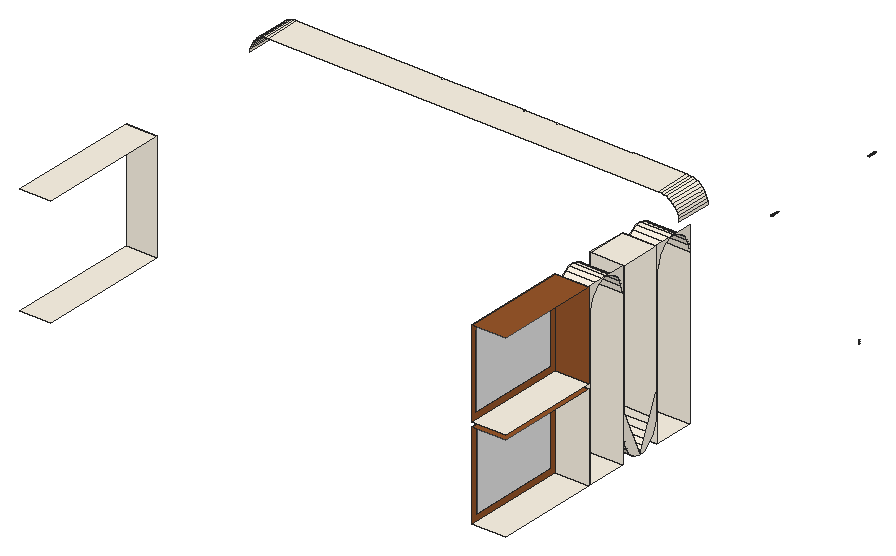
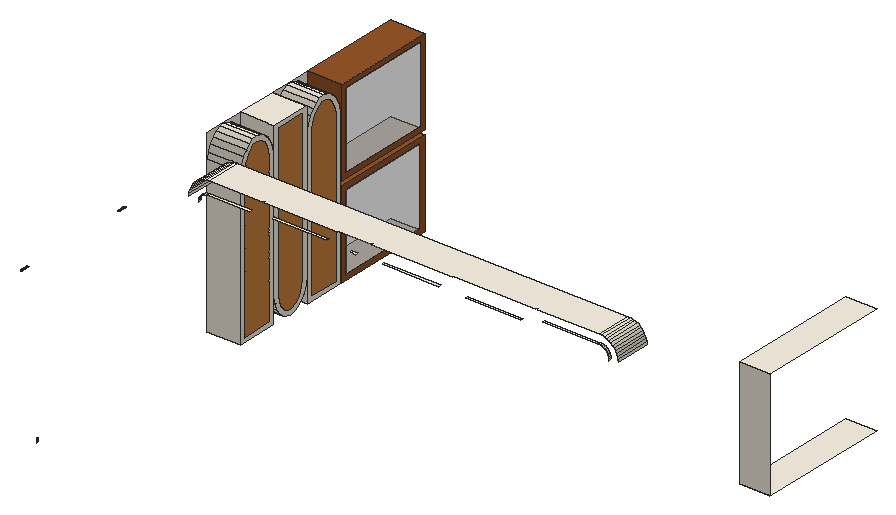
# SketchUp Ruby script. Lengths in inches.
U = 1.inch
M = Sketchup.active_model
def pt(a) = Geom::Point3d.new(a.map { |v| v * U })
def face(e, loops, mat)
  f = e.add_face(loops[0].map { |a| pt(a) })
  loops[1..].each { |l| e.add_face(l.map { |a| pt(a) }).erase! }
  f.material = f.back_material = mat if mat
  f
end
# faces: each face lists its corners as indices into pts; further lists are holes
def faces(e, pts, list, mat = nil) = list.each { |f| face(e, (f[0].is_a?(Array) ? f : [f]).map { |l| l.map { |i| pts[i] } }, mat) }
# xy, xz, yz: faces in a plane at the given z, y or x. An outline is a flat list of corners, or four numbers for a rectangle; further outlines are holes
def ring(l) = l.size == 4 ? [[l[0], l[1]], [l[2], l[1]], [l[2], l[3]], [l[0], l[3]]] : l.each_slice(2).to_a
def flat(e, list, mat, &to3) = list.each { |f| face(e, (f[0].is_a?(Array) ? f : [f]).map { |l| ring(l).map { |u, v| to3.(u, v) } }, mat) }
def xy(e, z, list, mat = nil) = flat(e, list, mat) { |x, y| [x, y, z] }
def xz(e, y, list, mat = nil) = flat(e, list, mat) { |x, z| [x, y, z] }
def yz(e, x, list, mat = nil) = flat(e, list, mat) { |y, z| [x, y, z] }
def lines(e, pts, list) = list.each { |a, b| e.add_line(pt(pts[a]), pt(pts[b])) }
# prism: a flat outline (further loops are holes) pulled along v
def prism(e, loops, v, mat = nil)
  f = face(e, loops, mat); d = Geom::Vector3d.new(v.map { |x| x * U })
  f.pushpull(f.normal.samedirection?(d) ? d.length : -d.length)
end
def box(e, o, s, mat = nil) = prism(e, [[o, [o[0] + s[0], o[1], o[2]], [o[0] + s[0], o[1] + s[1], o[2]], [o[0], o[1] + s[1], o[2]]]], [0, 0, s[2]], mat)
def at(x, y, z, deg = 0) = Geom::Transformation.translation(pt([x, y, z])) * Geom::Transformation.rotation(ORIGIN, Z_AXIS, deg.degrees)
def axes(o, x, y, z) = Geom::Transformation.new([*x, 0, *y, 0, *z, 0, *pt(o).to_a, 1])
def part(name) = M.definitions.add(name)
# library, detail: a bought-in or finely detailed component or shape, given as its bounding box
def library(name, o, s) = part(name).tap { |d| box(d.entities, o, s) }
def detail(e, o, s) = box(e.add_group.entities, o, s)
def put(e, d, t, mat = nil) = e.add_instance(d, t).tap { |i| i.material = mat if mat }
def group(e, t, mat = nil) = e.add_group.tap { |g| g.transformation = t; g.material = mat if mat }.entities
root = M.entities
M.materials.add("Material \#0").color = [86, 53, 35]
M.materials.add("Material \#1").color = [140, 140, 140]
M.materials.add("[0030_OldLace]").color = [253, 245, 230]
M.materials.add("[0040_Peru]").color = [205, 133, 63]
M.materials.add("[Translucent Glass Gray]").color = [128, 128, 128]
M.materials["[Translucent Glass Gray]"].alpha = 0.5
M.materials.add("[Wood Cherry Original]").color = [152, 86, 42]
c1 = part("3DGeom~17_Defintion")
yz(c1.entities,-1908.8,[[-436.03,-21.87,-436.73,-21.5,-435.91,-21.83],[436.03,-21.87,435.91,-21.83,436.73,-21.5],[-435.91,-21.83,-436.73,-21.5,-436.15,-21.125],[-435.91,-21.83,-436.15,-21.125,-435.87,-21.72],[435.91,-21.83,435.87,-21.72,436.15,-21.125],
  [435.91,-21.83,436.15,-21.125,436.73,-21.5],[-436.73,-21.5,-484.73,-21.37,-436.15,-1.11],[-471.46,-21.5,-484.73,-21.37,-436.73,-21.5],[-477.2,-21.5,-484.73,-21.37,-471.46,-21.5],[-481.82,-21.5,-484.73,-21.37,-477.2,-21.5],
  [-436.73,-21.5,-436.15,-1.11,-436.15,-21.125],[436.73,-21.5,436.15,-21.125,471.46,-21.5],[471.46,-21.5,436.15,-21.125,477.2,-21.5],[477.2,-21.5,436.15,-21.125,499.98,-0.85],[477.2,-21.5,499.98,-0.85,481.82,-21.5],
  [481.82,-21.5,487.35,-21,484.73,-21.37],[481.82,-21.5,491.8,-19.52,487.35,-21],[481.82,-21.5,497.64,-13.67,491.8,-19.52],[481.82,-21.5,499.98,-0.85,497.64,-13.67],[-484.73,-21.37,-498.5,-11.58,-499.84,-0.37],
  [-484.73,-21.37,-499.84,-0.37,-499.4,-0.5],[-484.73,-21.37,-499.4,-0.5,-436.15,-1.11],[-484.73,-21.37,-493.63,-18.42,-498.5,-11.58],[-484.73,-21.37,-489.71,-20.375,-493.63,-18.42],[-484.73,-21.37,-487.35,-21,-489.71,-20.375],
  [436.15,-21.125,436.15,-1.11,436.73,-0.74],[436.15,-21.125,436.73,-0.74,499.98,-0.85],[487.35,-21,491.8,-19.52,489.71,-20.375],[-489.71,-20.375,-491.8,-19.52,-493.63,-18.42],[491.8,-19.52,495.21,-17.08,493.63,-18.42],
  [491.8,-19.52,497.64,-13.67,495.21,-17.08],[-493.63,-18.42,-496.54,-15.5,-498.5,-11.58],[-493.63,-18.42,-495.21,-17.08,-496.54,-15.5],[495.21,-17.08,497.64,-13.67,496.54,-15.5],[-496.54,-15.5,-497.64,-13.67,-498.5,-11.58],
  [497.64,-13.67,499.125,-9.22,498.5,-11.58],[497.64,-13.67,499.625,-3.69,499.125,-9.22],[497.64,-13.67,499.98,-0.85,499.625,-3.69],[-498.5,-11.58,-499.625,-3.69,-499.84,-0.37],[-498.5,-11.58,-499.5,-6.6,-499.625,-3.69],
  [-498.5,-11.58,-499.125,-9.22,-499.5,-6.6],[499.125,-9.22,499.625,-3.69,499.5,-6.6],[-499.625,-3.69,-499.98,-0.85,-500,-0.52],[-499.625,-3.69,-500,-0.52,-499.84,-0.37],[-436.15,-1.11,-499.4,-0.5,-471.46,-0.74],
  [-436.15,-1.11,-471.46,-0.74,-436.73,-0.74],[-436.15,-1.11,-436.73,-0.74,-435.91,-0.41],[-436.15,-1.11,-435.91,-0.41,-435.87,-0.52],[436.15,-1.11,435.87,-0.52,435.91,-0.41],[436.15,-1.11,435.91,-0.41,436.73,-0.74],
  [499.98,-0.85,436.73,-0.74,471.46,-0.74],[499.98,-0.85,471.46,-0.74,499.4,-0.5],[499.98,-0.85,499.4,-0.5,499.96,-0.41],[499.98,-0.85,499.96,-0.41,500,-0.52],[-436.73,-0.74,-436.03,-0.37,-435.91,-0.41],
  [436.73,-0.74,435.91,-0.41,436.03,-0.37],[-500,-0.52,-499.96,-0.41,-499.84,-0.37],[499.4,-0.5,499.84,-0.37,499.96,-0.41],[-499.84,141.21,-499.96,141.25,-499.4,141.35],[-436.03,141.21,-436.73,141.59,-435.91,141.25],
  [436.03,141.21,435.91,141.25,436.73,141.59],[499.84,141.21,484.73,162.21,498.5,152.42],[499.84,141.21,499.4,141.35,484.73,162.21],[499.84,141.21,498.5,152.42,499.625,144.53],[499.84,141.21,499.625,144.53,500,141.37],
  [499.84,141.21,500,141.37,499.96,141.25],[-499.96,141.25,-500,141.37,-499.98,141.69],[-499.96,141.25,-499.98,141.69,-499.4,141.35],[-435.91,141.25,-436.73,141.59,-436.15,141.96],[-435.91,141.25,-436.15,141.96,-435.87,141.37],
  [435.91,141.25,435.87,141.37,436.15,141.96],[435.91,141.25,436.15,141.96,436.73,141.59],[-499.4,141.35,-499.98,141.69,-471.46,141.59],[499.4,141.35,436.15,141.96,484.73,162.21],[499.4,141.35,471.46,141.59,436.15,141.96],
  [500,141.37,499.625,144.53,499.98,141.69],[-436.73,141.59,-499.98,141.69,-436.15,161.97],[-471.46,141.59,-499.98,141.69,-436.73,141.59],[-436.73,141.59,-436.15,161.97,-436.15,141.96],[436.73,141.59,436.15,141.96,471.46,141.59],
  [-499.98,141.69,-477.2,162.34,-436.15,161.97],[-499.98,141.69,-481.82,162.34,-477.2,162.34],[-499.98,141.69,-497.64,154.51,-481.82,162.34],[-499.98,141.69,-499.625,144.53,-497.64,154.51],[436.15,141.96,436.15,161.97,436.73,162.34],
  [436.15,141.96,436.73,162.34,484.73,162.21],[-499.625,144.53,-499.125,150.07,-497.64,154.51],[-499.625,144.53,-499.5,147.44,-499.125,150.07],[499.625,144.53,498.5,152.42,499.5,147.44],[499.5,147.44,498.5,152.42,499.125,150.07],
  [-499.125,150.07,-498.5,152.42,-497.64,154.51],[498.5,152.42,484.73,162.21,493.63,159.26],[498.5,152.42,493.63,159.26,496.54,156.34],[498.5,152.42,496.54,156.34,497.64,154.51],[-497.64,154.51,-491.8,160.36,-481.82,162.34],
  [-497.64,154.51,-495.21,157.92,-491.8,160.36],[-497.64,154.51,-496.54,156.34,-495.21,157.92],[496.54,156.34,493.63,159.26,495.21,157.92],[-495.21,157.92,-493.63,159.26,-491.8,160.36],[493.63,159.26,484.73,162.21,489.71,161.22],
  [493.63,159.26,489.71,161.22,491.8,160.36],[-491.8,160.36,-487.35,161.84,-481.82,162.34],[-491.8,160.36,-489.71,161.22,-487.35,161.84],[489.71,161.22,484.73,162.21,487.35,161.84],[-487.35,161.84,-484.73,162.21,-481.82,162.34],
  [-436.15,161.97,-477.2,162.34,-471.46,162.34],[-436.15,161.97,-471.46,162.34,-436.73,162.34],[-436.15,161.97,-436.73,162.34,-435.91,162.68],[-436.15,161.97,-435.91,162.68,-435.87,162.56],[436.15,161.97,435.87,162.56,435.91,162.68],
  [436.15,161.97,435.91,162.68,436.73,162.34],[484.73,162.21,436.73,162.34,471.46,162.34],[484.73,162.21,471.46,162.34,477.2,162.34],[484.73,162.21,477.2,162.34,481.82,162.34],[-436.73,162.34,-436.03,162.72,-435.91,162.68],
  [436.73,162.34,435.91,162.68,436.03,162.72]],"Material \#0")
xy(root,61.5362,[[143,315.4649,153,346.4649],[143,346.9649,153,358.9649],[143,371.9649,153,383.9649]],"[0030_OldLace]")
xy(root,63.5,[[0,326.0274,9,365.5274]],"[0030_OldLace]")
xy(root,87.4225,[[143,315.4649,153,346.4649]],"[Wood Cherry Original]")
xy(root,88.8265,[[143,315.4649,153,346.4649]],"[0030_OldLace]")
xy(root,96,[[0,326.0274,9,365.5274]],"[0030_OldLace]")
xy(root,111.1281,[[44.5074,402.0274,61.0233,402.7149]],"[0030_OldLace]")
xy(root,111.275,[[93.6625,402.0274,95.344,402.7149]],"[0030_OldLace]")
xy(root,111.4014,[[68.9818,402.0274,85.7849,402.7149]],"[0030_OldLace]")
xy(root,111.6138,[[125.3337,402.0274,137.8631,402.7149]],"[0030_OldLace]")
xy(root,112.1331,[[102.4294,402.0274,118.5869,402.7149]],"[0030_OldLace]")
xy(root,112.8044,[[21.5933,402.0274,37.9421,402.7149]],"[0030_OldLace]")
xy(root,114.625,[[143,359.4649,153,371.4649]],"[0030_OldLace]")
xy(root,114.625,[[143,315.4649,153,346.4649]],"[Wood Cherry Original]")
xy(root,115,[[21.5933,391.4649,137.8631,391.4649,137.8631,402.0274,121.9475,402.0274,121.9475,401.4649,121.4538,401.4649,121.4538,402.0274,99.5625,402.0274,99.5625,401.4649,99.069,401.4649,99.069,402.0274,89.9375,402.0274,89.9375,401.4649,89.3836,401.4649,89.3836,402.0274,65.3832,402.0274,65.3832,401.4649,64.8952,401.4649,64.8952,402.0274,40.6355,402.0274,40.6355,401.4649,40.1377,401.4649,40.1377,402.0274,21.5933,402.0274]],"[0030_OldLace]")
xz(root,346.4649,[[143,61.5362,153,87.4225]],"[0030_OldLace]")
xz(root,346.4649,[[143,88.8265,153,114.625]],"[Wood Cherry Original]")
xz(root,346.9649,[[143,61.5362,153,107.605]],"[0030_OldLace]")
xz(root,358.9649,[[143,61.5362,153,107.605]],"[0030_OldLace]")
xz(root,359.4649,[[143,68.5562,153,114.625]],"[0030_OldLace]")
xz(root,365.5274,[[0,63.5,9,96]],"[0030_OldLace]")
xz(root,371.4649,[[143,68.5562,153,114.625]],"[0030_OldLace]")
xz(root,371.9649,[[143,61.5362,153,107.605]],"[0030_OldLace]")
xz(root,383.9649,[[143,61.5362,153,107.605]],"[0030_OldLace]")
yz(root,143,[[[346.9649,61.5362,346.9649,107.605,347.3775,109.4972,348.0885,111.2059,349.0598,112.64,350.2396,113.7227,351.5649,114.3964,352.9649,114.625,354.3649,114.3964,355.6902,113.7227,356.87,112.64,357.8413,111.2059,358.5523,109.4972,358.9649,107.605,358.9649,61.5362],[348.1935,62.7649,357.7363,62.7649,357.7363,107.4726,357.3754,109.1274,356.7546,110.6195,355.9334,111.8319,354.9835,112.7037,353.9784,113.2146,352.9649,113.3801,351.9514,113.2146,350.9463,112.7037,349.9964,111.8319,349.1752,110.6195,348.5544,109.1274,348.1935,107.4726]],[[365.4649,61.5362,364.0649,61.7649,362.7396,62.4385,361.5598,63.5213,360.5885,64.9553,359.8775,66.664,359.4649,68.5562,359.4649,114.625,371.4649,114.625,371.4649,68.5562,371.0523,66.664,370.3413,64.9553,369.37,63.5213,368.1902,62.4385,366.8649,61.7649],[365.4649,62.7593,366.4852,62.9259,367.4959,63.4396,368.4498,64.3151,369.2737,65.5314,369.8961,67.0274,370.2579,68.6863,370.2579,113.418,360.6719,113.418,360.6719,68.6863,361.0337,67.0274,361.6561,65.5314,362.48,64.3151,363.4339,63.4396,364.4446,62.9259]],[[371.9649,61.5362,371.9649,107.605,372.3775,109.4972,373.0885,111.2059,374.0598,112.64,375.2396,113.7227,376.5649,114.3964,377.9649,114.625,379.3649,114.3964,380.6902,113.7227,381.87,112.64,382.8413,111.2059,383.5523,109.4972,383.9649,107.605,383.9649,61.5362],[373.3454,62.9167,382.5844,62.9167,382.5844,107.4562,382.23,109.0817,381.6203,110.5471,380.8176,111.7321,379.8961,112.5778,378.9307,113.0685,377.9649,113.2263,376.9991,113.0685,376.0337,112.5778,375.1122,111.7321,374.3095,110.5471,373.6998,109.0817,373.3454,107.4562]]],"[0030_OldLace]")
yz(root,143,[[365.4649,62.7593,364.4446,62.9259,363.4339,63.4396,362.48,64.3151,361.6561,65.5314,361.0337,67.0274,360.6719,68.6863,360.6719,113.418,370.2579,113.418,370.2579,68.6863,369.8961,67.0274,369.2737,65.5314,368.4498,64.3151,367.4959,63.4396,366.4852,62.9259],[348.1935,62.7649,348.1935,107.4726,348.5544,109.1274,349.1752,110.6195,349.9964,111.8319,350.9463,112.7037,351.9514,113.2146,352.9649,113.3801,353.9784,113.2146,354.9835,112.7037,355.9334,111.8319,356.7546,110.6195,357.3754,109.1274,357.7363,107.4726,357.7363,62.7649],[373.3454,62.9167,373.3454,107.4562,373.6998,109.0817,374.3095,110.5471,375.1122,111.7321,376.0337,112.5778,376.9991,113.0685,377.9649,113.2263,378.9307,113.0685,379.8961,112.5778,380.8176,111.7321,381.6203,110.5471,382.23,109.0817,382.5844,107.4562,382.5844,62.9167]],"[0040_Peru]")
yz(root,143,[[317.1079,63.1792,344.8219,85.7795],[317.022,90.3836,344.9078,113.0679]],"[Translucent Glass Gray]")
yz(root,143,[[[315.4649,61.5362,346.4649,87.4225],[317.1079,63.1792,344.8219,85.7795]],[[315.4649,88.8265,346.4649,114.625],[317.022,90.3836,344.9078,113.0679]]],"[Wood Cherry Original]")
yz(root,153,[[365.4649,61.5362,364.0649,61.7649,362.7396,62.4385,361.5598,63.5213,360.5885,64.9553,359.8775,66.664,359.4649,68.5562,359.4649,75.3],[365.4649,61.5362,371.4649,75.3,371.4649,68.5562,371.0523,66.664,370.3413,64.9553,369.37,63.5213,368.1902,62.4385,366.8649,61.7649],[346.9649,107.605,346.9649,114.625,352.9649,114.625,351.5649,114.3964,350.2396,113.7227,349.0598,112.64,348.0885,111.2059,347.3775,109.4972],[358.9649,107.605,358.5523,109.4972,357.8413,111.2059,356.87,112.64,355.6902,113.7227,354.3649,114.3964,352.9649,114.625,358.9649,114.625],[371.9649,107.605,371.9649,114.625,377.9649,114.625,376.5649,114.3964,375.2396,113.7227,374.0598,112.64,373.0885,111.2059,372.3775,109.4972],
  [383.9649,107.605,383.5523,109.4972,382.8413,111.2059,381.87,112.64,380.6902,113.7227,379.3649,114.3964,377.9649,114.625,383.9649,114.625]],"[0030_OldLace]")
yz(root,155.6343,[[444.0231,57.4405,443.928,57.5113,443.8319,57.5685],[444.0231,57.4405,443.9154,57.4752,443.967,57.4495],[444.0231,57.4405,443.9736,57.4886,443.928,57.5113],[443.9154,57.4752,443.8319,57.5685,443.8698,57.5155],[443.7802,57.827,443.8775,58.059,443.8738,58.0531],
  [443.7802,57.827,443.8806,58.0652,443.8775,58.059],[443.8288,57.9145,443.8544,57.9704,443.8806,58.0652],[443.8544,57.9704,443.8847,58.0789,443.8806,58.0652],[443.8544,57.9704,443.8879,58.0171,443.8847,58.0789],[443.8879,58.0171,443.8861,58.0949,443.8847,58.0789],
  [443.8879,58.0171,443.8861,58.46,443.8861,58.0949],[443.8879,58.0171,443.928,58.0527,443.8861,58.46],[443.928,58.0527,443.9736,58.0754,443.8861,58.46],[443.8806,58.0652,443.8847,58.0789,443.883,58.0718],[443.9736,58.0754,444.0231,58.0834,443.8861,58.46],
  [443.8847,58.0789,443.8861,58.0949,443.8858,58.0866],[444.0231,58.0834,443.9163,58.5794,443.8861,58.46],[443.8861,58.46,443.9163,58.5794,443.8898,58.5038],[443.8898,58.5038,443.9163,58.5794,443.9001,58.5439],[443.9163,58.5794,443.9629,58.6315,443.9375,58.609],
  [443.9163,58.5794,444.0231,58.6509,443.9629,58.6315],[443.9629,58.6315,444.0231,58.6509,443.9917,58.6459]],"Material \#1")
p = [[153,365.4649,61.5362],[153,364.0649,61.7649],[143,364.0649,61.7649],[143,365.4649,61.5362],[153,366.8649,61.7649],[143,366.8649,61.7649],
  [153,362.7396,62.4385],[143,362.7396,62.4385],[153,368.1902,62.4385],[143,368.1902,62.4385],[153,361.5598,63.5213],[143,361.5598,63.5213],
  [153,369.37,63.5213],[143,369.37,63.5213],[153,360.5885,64.9553],[143,360.5885,64.9553],[153,370.3413,64.9553],[143,370.3413,64.9553],
  [153,359.8775,66.664],[143,359.8775,66.664],[153,371.0523,66.664],[143,371.0523,66.664],[153,359.4649,68.5562],[143,359.4649,68.5562],
  [153,371.4649,68.5562],[143,371.4649,68.5562],[153,346.9649,107.605],[153,347.3775,109.4972],[143,347.3775,109.4972],[143,346.9649,107.605],
  [153,358.5523,109.4972],[153,358.9649,107.605],[143,358.9649,107.605],[143,358.5523,109.4972],[153,371.9649,107.605],[153,372.3775,109.4972],
  [143,372.3775,109.4972],[143,371.9649,107.605],[153,383.5523,109.4972],[153,383.9649,107.605],[143,383.9649,107.605],[143,383.5523,109.4972],
  [143.8855,391.4649,109.7185],[143.9375,391.4649,108.9256],[143.9375,402.0274,108.9256],[143.8855,402.0274,109.7185],[140.5283,402.0274,109.2765],[140.5513,402.0274,108.9256],
  [140.5513,402.7149,108.9256],[140.5283,402.7149,109.2765],[140.4597,402.0274,109.6214],[140.4597,402.7149,109.6214],[153,348.0885,111.2059],[143,348.0885,111.2059],
  [153,357.8413,111.2059],[143,357.8413,111.2059],[153,373.0885,111.2059],[143,373.0885,111.2059],[153,382.8413,111.2059],[143,382.8413,111.2059],
  [16.0477,391.4649,109.4544],[16.0952,391.4649,110.1782],[16.0952,402.0274,110.1782],[16.0477,402.0274,109.4544],[18.2433,402.0274,109.4544],[18.272,402.0274,109.8916],
  [18.272,402.7149,109.8916],[18.2433,402.7149,109.4544],[140.3467,402.0274,109.9544],[140.3467,402.7149,109.9544],[143.7305,391.4649,110.4978],[143.7305,402.0274,110.4978],
  [18.3575,402.0274,110.3214],[18.3575,402.7149,110.3214],[140.1911,402.0274,110.2697],[140.1911,402.7149,110.2697],[16.2367,391.4649,110.8897],[16.2367,402.0274,110.8897],
  [18.4983,402.0274,110.7364],[18.4983,402.7149,110.7364],[139.9958,402.0274,110.5621],[139.9958,402.7149,110.5621],[143.4751,391.4649,111.2502],[143.4751,402.0274,111.2502],
  [139.764,402.0274,110.8265],[139.764,402.7149,110.8265],[18.6921,402.0274,111.1294],[18.6921,402.7149,111.1294],[139.4996,402.0274,111.0583],[139.4996,402.7149,111.0583],
  [16.4698,391.4649,111.5766],[16.4698,402.0274,111.5766],[18.9356,402.0274,111.4937],[18.9356,402.7149,111.4937],[139.2072,402.0274,111.2536],[139.2072,402.7149,111.2536],
  [153,349.0598,112.64],[143,349.0598,112.64],[153,356.87,112.64],[143,356.87,112.64],[153,374.0598,112.64],[143,374.0598,112.64],
  [153,381.87,112.64],[143,381.87,112.64],[143.1237,391.4649,111.9628],[143.1237,402.0274,111.9628],[138.8919,402.0274,111.4092],[138.8919,402.7149,111.4092],
  [138.5589,402.0274,111.5222],[138.5589,402.7149,111.5222],[19.2245,402.0274,111.8232],[19.2245,402.7149,111.8232],[138.214,402.0274,111.5908],[138.214,402.7149,111.5908],
  [16.7907,391.4649,112.2272],[16.7907,402.0274,112.2272],[137.8631,402.0274,111.6138],[137.8631,402.7149,111.6138],[19.554,402.0274,112.1121],[19.554,402.7149,112.1121],
  [142.6823,391.4649,112.6235],[142.6823,402.0274,112.6235],[19.9183,402.0274,112.3556],[19.9183,402.7149,112.3556],[17.1937,391.4649,112.8303],[17.1937,402.0274,112.8303],
  [20.3113,402.0274,112.5494],[20.3113,402.7149,112.5494],[20.7263,402.0274,112.6902],[20.7263,402.7149,112.6902],[153,350.2396,113.7227],[143,350.2396,113.7227],
  [153,355.6902,113.7227],[143,355.6902,113.7227],[153,375.2396,113.7227],[143,375.2396,113.7227],[153,380.6902,113.7227],[143,380.6902,113.7227],
  [142.1584,391.4649,113.2209],[142.1584,402.0274,113.2209],[21.1561,402.0274,112.7757],[21.1561,402.7149,112.7757],[17.672,391.4649,113.3757],[17.672,402.0274,113.3757],
  [21.5933,402.0274,112.8044],[21.5933,402.7149,112.8044],[141.561,391.4649,113.7448],[141.561,402.0274,113.7448],[18.2174,391.4649,113.854],[18.2174,402.0274,113.854],
  [153,351.5649,114.3964],[143,351.5649,114.3964],[153,354.3649,114.3964],[143,354.3649,114.3964],[153,376.5649,114.3964],[143,376.5649,114.3964],
  [153,379.3649,114.3964],[143,379.3649,114.3964],[140.9003,391.4649,114.1862],[140.9003,402.0274,114.1862],[18.8205,391.4649,114.257],[18.8205,402.0274,114.257],
  [140.1877,391.4649,114.5376],[140.1877,402.0274,114.5376],[19.4711,391.4649,114.5779],[19.4711,402.0274,114.5779],[153,352.9649,114.625],[143,352.9649,114.625],
  [153,377.9649,114.625],[143,377.9649,114.625],[139.4353,391.4649,114.793],[139.4353,402.0274,114.793],[20.158,391.4649,114.811],[20.158,402.0274,114.811],
  [20.8695,391.4649,114.9526],[20.8695,402.0274,114.9526],[138.656,391.4649,114.948],[138.656,402.0274,114.948],[137.8631,391.4649,115],[137.8631,402.0274,115],
  [21.5933,391.4649,115],[21.5933,402.0274,115]]
faces(root,p,[[0,1,2,3],[4,0,3,5],[1,6,7,2],[8,4,5,9],[6,10,11,7],[12,8,9,13],[10,14,15,11],[16,12,13,17],
  [14,18,19,15],[20,16,17,21],[18,22,23,19],[24,20,21,25],[26,27,28,29],[30,31,32,33],[34,35,36,37],[38,39,40,41],
  [42,43,44,45],[46,47,48,49],[50,46,49,51],[27,52,53,28],[54,30,33,55],[35,56,57,36],[58,38,41,59],[60,61,62,63],
  [64,65,66,67],[68,50,51,69],[70,42,45,71],[65,72,73,66],[74,68,69,75],[61,76,77,62],[72,78,79,73],[80,74,75,81],
  [82,70,71,83],[84,80,81,85],[78,86,87,79],[88,84,85,89],[76,90,91,77],[86,92,93,87],[94,88,89,95],[52,96,97,53],
  [98,54,55,99],[56,100,101,57],[102,58,59,103],[104,82,83,105],[106,94,95,107],[108,106,107,109],[92,110,111,93],[112,108,109,113],
  [90,114,115,91],[116,112,113,117],[110,118,119,111],[120,104,105,121],[118,122,123,119],[114,124,125,115],[122,126,127,123],[126,128,129,127],
  [96,130,131,97],[132,98,99,133],[100,134,135,101],[136,102,103,137],[138,120,121,139],[128,140,141,129],[124,142,143,125],[140,144,145,141],
  [146,138,139,147],[142,148,149,143],[130,150,151,131],[152,132,133,153],[134,154,155,135],[156,136,137,157],[158,146,147,159],[148,160,161,149],
  [162,158,159,163],[160,164,165,161],[150,166,167,151],[166,152,153,167],[154,168,169,155],[168,156,157,169],[170,162,163,171],[164,172,173,165],
  [172,174,175,173],[176,170,171,177],[178,176,177,179],[174,180,181,175]],"[0030_OldLace]")
put(root,c1,axes([155.34,430.68,2.53],[0,0,-0.05421],[0,-0.03891,0],[0.00272,0,0]),"Material \#0")
